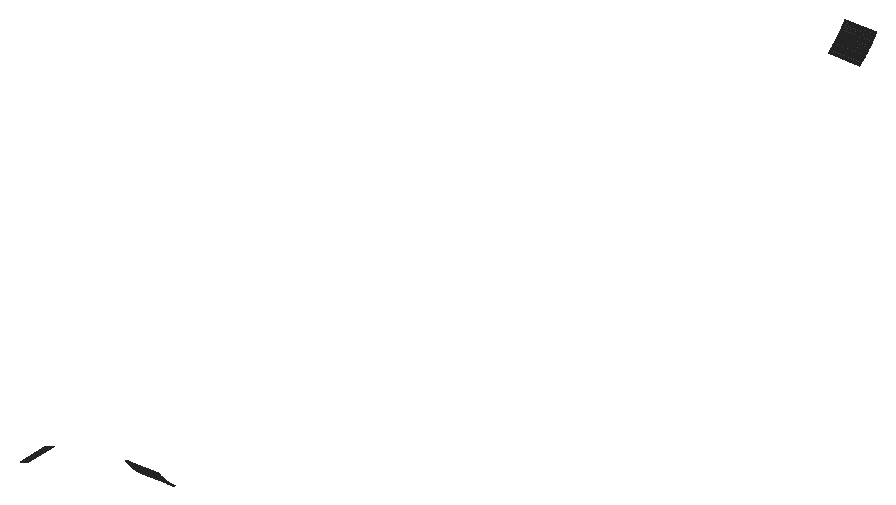
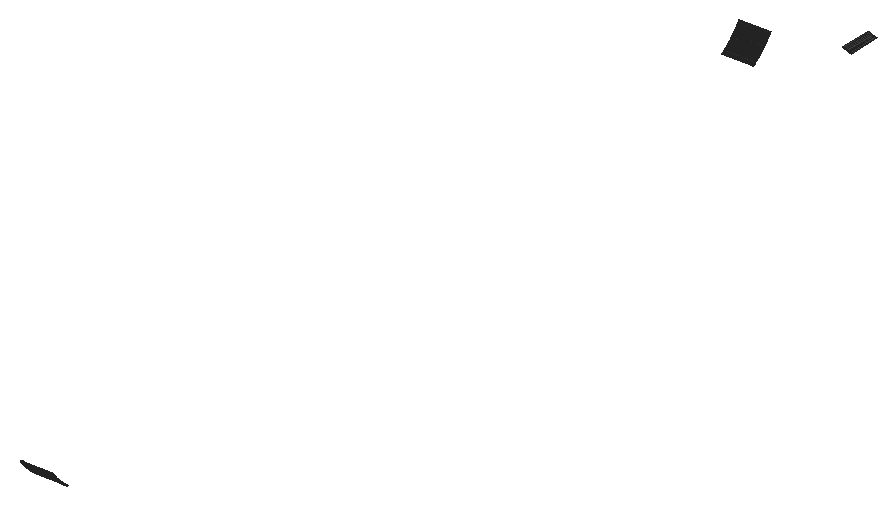
# SketchUp Ruby script. Lengths in inches.
U = 1.inch
M = Sketchup.active_model
def pt(a) = Geom::Point3d.new(a.map { |v| v * U })
def face(e, loops, mat)
  f = e.add_face(loops[0].map { |a| pt(a) })
  loops[1..].each { |l| e.add_face(l.map { |a| pt(a) }).erase! }
  f.material = f.back_material = mat if mat
  f
end
# faces: each face lists its corners as indices into pts; further lists are holes
def faces(e, pts, list, mat = nil) = list.each { |f| face(e, (f[0].is_a?(Array) ? f : [f]).map { |l| l.map { |i| pts[i] } }, mat) }
# xy, xz, yz: faces in a plane at the given z, y or x. An outline is a flat list of corners, or four numbers for a rectangle; further outlines are holes
def ring(l) = l.size == 4 ? [[l[0], l[1]], [l[2], l[1]], [l[2], l[3]], [l[0], l[3]]] : l.each_slice(2).to_a
def flat(e, list, mat, &to3) = list.each { |f| face(e, (f[0].is_a?(Array) ? f : [f]).map { |l| ring(l).map { |u, v| to3.(u, v) } }, mat) }
def xy(e, z, list, mat = nil) = flat(e, list, mat) { |x, y| [x, y, z] }
def xz(e, y, list, mat = nil) = flat(e, list, mat) { |x, z| [x, y, z] }
def yz(e, x, list, mat = nil) = flat(e, list, mat) { |y, z| [x, y, z] }
def lines(e, pts, list) = list.each { |a, b| e.add_line(pt(pts[a]), pt(pts[b])) }
# prism: a flat outline (further loops are holes) pulled along v
def prism(e, loops, v, mat = nil)
  f = face(e, loops, mat); d = Geom::Vector3d.new(v.map { |x| x * U })
  f.pushpull(f.normal.samedirection?(d) ? d.length : -d.length)
end
def box(e, o, s, mat = nil) = prism(e, [[o, [o[0] + s[0], o[1], o[2]], [o[0] + s[0], o[1] + s[1], o[2]], [o[0], o[1] + s[1], o[2]]]], [0, 0, s[2]], mat)
def at(x, y, z, deg = 0) = Geom::Transformation.translation(pt([x, y, z])) * Geom::Transformation.rotation(ORIGIN, Z_AXIS, deg.degrees)
def axes(o, x, y, z) = Geom::Transformation.new([*x, 0, *y, 0, *z, 0, *pt(o).to_a, 1])
def part(name) = M.definitions.add(name)
# library, detail: a bought-in or finely detailed component or shape, given as its bounding box
def library(name, o, s) = part(name).tap { |d| box(d.entities, o, s) }
def detail(e, o, s) = box(e.add_group.entities, o, s)
def put(e, d, t, mat = nil) = e.add_instance(d, t).tap { |i| i.material = mat if mat }
def group(e, t, mat = nil) = e.add_group.tap { |g| g.transformation = t; g.material = mat if mat }.entities
root = M.entities
M.materials.add("1432 AP 8245 TAR ROAD").color = [71, 72, 75]
p = [[573,122.21,150.67],[573,122.4375,150.5],[585,122.4375,150.5],[585,122.21,150.67],[573,121.98,150.83],[585,121.98,150.83],
  [573,452.53,150.67],[573,452.76,150.83],[585,452.76,150.83],[585,452.53,150.67],[573,121.75,151],[585,121.75,151],
  [573,452.99,151],[585,452.99,151],[573,121.53,151.17],[585,121.53,151.17],[573,453.21,151.17],[585,453.21,151.17],
  [573,121.31,151.35],[585,121.31,151.35],[573,453.43,151.35],[585,453.43,151.35],[573,121.08,151.52],[585,121.08,151.52],
  [573,453.66,151.52],[585,453.66,151.52],[573,120.86,151.7],[585,120.86,151.7],[573,453.88,151.7],[585,453.88,151.7],
  [573,120.64,151.875],[585,120.64,151.875],[573,454.1,151.875],[585,454.1,151.875],[573,120.42,152.05],[585,120.42,152.05],
  [573,454.32,152.05],[585,454.32,152.05],[573,120.21,152.23],[585,120.21,152.23],[573,454.53,152.23],[585,454.53,152.23],
  [573,119.99,152.42],[585,119.99,152.42],[573,454.75,152.42],[585,454.75,152.42],[573,119.78,152.6],[585,119.78,152.6],
  [573,454.96,152.6],[585,454.96,152.6],[573,119.5625,152.79],[585,119.5625,152.79],[573,455.18,152.79],[585,455.18,152.79],
  [573,119.35,152.98],[585,119.35,152.98],[573,455.39,152.98],[585,455.39,152.98],[573,119.14,153.17],[585,119.14,153.17],
  [573,455.6,153.17],[585,455.6,153.17],[573,118.93,153.36],[585,118.93,153.36],[573,455.81,153.36],[585,455.81,153.36],
  [573,118.73,153.55],[585,118.73,153.55],[573,456.01,153.55],[585,456.01,153.55],[573,118.52,153.74],[585,118.52,153.74],
  [573,456.22,153.74],[585,456.22,153.74],[573,118.32,153.94],[585,118.32,153.94],[573,456.42,153.94],[585,456.42,153.94],
  [573,118.11,154.14],[585,118.11,154.14],[573,456.625,154.14],[585,456.625,154.14],[573,117.91,154.34],[585,117.91,154.34],
  [573,456.83,154.34],[585,456.83,154.34],[573,117.71,154.54],[585,117.71,154.54],[573,457.02,154.54],[585,457.02,154.54],
  [573,117.52,154.74],[585,117.52,154.74],[573,457.22,154.74],[585,457.22,154.74],[573,117.32,154.94],[585,117.32,154.94],
  [573,457.42,154.94],[585,457.42,154.94],[573,117.13,155.15],[585,117.13,155.15],[573,457.61,155.15],[585,457.61,155.15],
  [573,116.93,155.36],[585,116.93,155.36],[573,457.81,155.36],[585,457.81,155.36],[573,116.74,155.5625],[585,116.74,155.5625],
  [573,458,155.5625],[585,458,155.5625],[573,116.55,155.77],[585,116.55,155.77],[573,458.1875,155.77],[585,458.1875,155.77],
  [573,116.37,155.98],[585,116.37,155.98],[573,458.375,155.98],[585,458.375,155.98],[573,116.18,156.2],[585,116.18,156.2],
  [573,458.56,156.2],[585,458.56,156.2],[573,116,156.41],[585,116,156.41],[573,458.74,156.41],[585,458.74,156.41],
  [573,115.8125,156.63],[585,115.8125,156.63],[573,458.93,156.63],[585,458.93,156.63],[573,115.63,156.84],[585,115.63,156.84],
  [573,459.11,156.84],[585,459.11,156.84],[573,115.45,157.0625],[585,115.45,157.0625],[573,459.29,157.0625],[585,459.29,157.0625],
  [573,115.27,157.28],[585,115.27,157.28],[573,459.47,157.28],[585,459.47,157.28],[547.31,107.37,157.3],[547.59,107.37,157.38],
  [547.59,95.37,157.38],[547.31,95.37,157.3],[573,115.1,157.5],[585,115.1,157.5],[573,459.64,157.5],[585,459.64,157.5],
  [547.86,107.37,157.47],[547.86,95.37,157.47],[548.125,107.37,157.55],[548.125,95.37,157.55],[573,114.92,157.73],[585,114.92,157.73],
  [573,459.82,157.73],[585,459.82,157.73],[548.39,107.37,157.64],[548.39,95.37,157.64],[548.66,107.37,157.73],[548.66,95.37,157.73],
  [548.93,107.37,157.83],[548.93,95.37,157.83],[573,114.75,157.95],[585,114.75,157.95],[573,459.99,157.95],[585,459.99,157.95],
  [549.19,107.37,157.92],[549.19,95.37,157.92],[549.46,107.37,158.02],[549.46,95.37,158.02],[549.73,107.37,158.12],[549.73,95.37,158.12],
  [573,114.58,158.18],[585,114.58,158.18],[573,460.16,158.18],[585,460.16,158.18],[549.99,107.37,158.22],[549.99,95.37,158.22],
  [550.25,107.37,158.32],[550.25,95.37,158.32],[573,114.41,158.4],[585,114.41,158.4],[573,460.33,158.4],[585,460.33,158.4],
  [550.51,107.37,158.43],[550.51,95.37,158.43],[573,114.25,158.63],[585,114.25,158.63],[573,460.49,158.63],[585,460.49,158.63]]
faces(root,p,[[0,1,2,3],[4,0,3,5],[6,7,8,9],[10,4,5,11],[7,12,13,8],[14,10,11,15],[12,16,17,13],[18,14,15,19],
  [16,20,21,17],[22,18,19,23],[20,24,25,21],[26,22,23,27],[24,28,29,25],[30,26,27,31],[28,32,33,29],[34,30,31,35],
  [32,36,37,33],[38,34,35,39],[36,40,41,37],[42,38,39,43],[40,44,45,41],[46,42,43,47],[44,48,49,45],[50,46,47,51],
  [48,52,53,49],[54,50,51,55],[52,56,57,53],[58,54,55,59],[56,60,61,57],[62,58,59,63],[60,64,65,61],[66,62,63,67],
  [64,68,69,65],[70,66,67,71],[68,72,73,69],[74,70,71,75],[72,76,77,73],[78,74,75,79],[76,80,81,77],[82,78,79,83],
  [80,84,85,81],[86,82,83,87],[84,88,89,85],[90,86,87,91],[88,92,93,89],[94,90,91,95],[92,96,97,93],[98,94,95,99],
  [96,100,101,97],[102,98,99,103],[100,104,105,101],[106,102,103,107],[104,108,109,105],[110,106,107,111],[108,112,113,109],[114,110,111,115],
  [112,116,117,113],[118,114,115,119],[116,120,121,117],[122,118,119,123],[120,124,125,121],[126,122,123,127],[124,128,129,125],[130,126,127,131],
  [128,132,133,129],[134,130,131,135],[132,136,137,133],[138,134,135,139],[136,140,141,137],[142,143,144,145],[146,138,139,147],[140,148,149,141],
  [143,150,151,144],[150,152,153,151],[154,146,147,155],[148,156,157,149],[152,158,159,153],[158,160,161,159],[160,162,163,161],[164,154,155,165],
  [156,166,167,157],[162,168,169,163],[168,170,171,169],[170,172,173,171],[174,164,165,175],[166,176,177,167],[172,178,179,173],[178,180,181,179],
  [182,174,175,183],[176,184,185,177],[180,186,187,181],[188,182,183,189],[184,190,191,185]],"1432 AP 8245 TAR ROAD")
